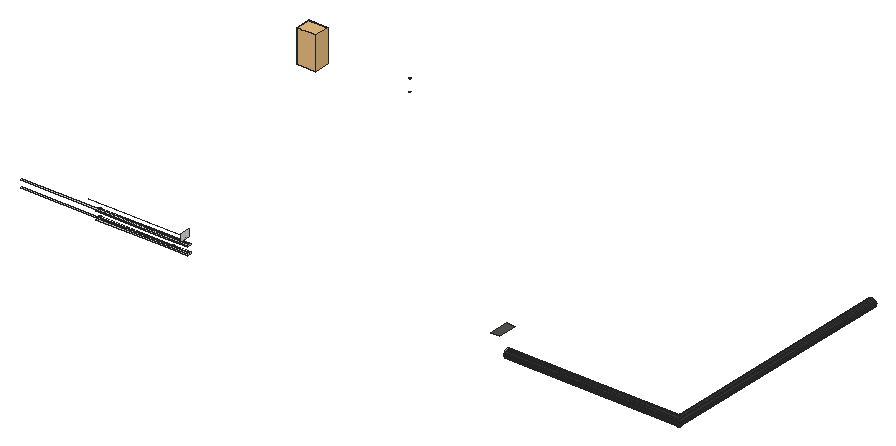
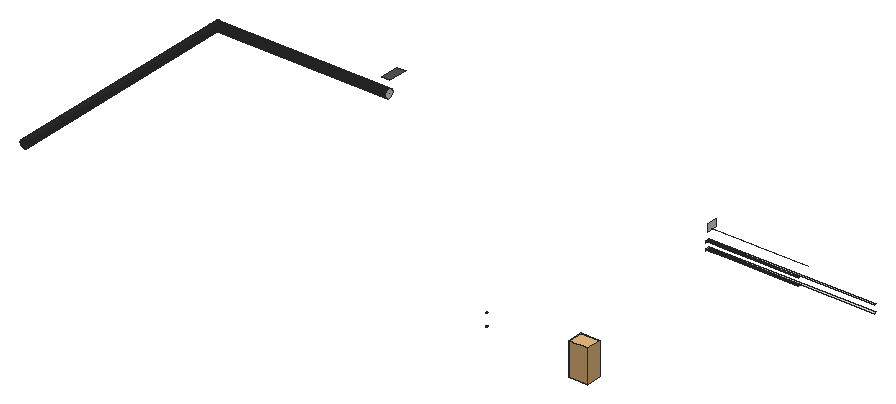
# SketchUp Ruby script. Lengths in inches.
U = 1.inch
M = Sketchup.active_model
def pt(a) = Geom::Point3d.new(a.map { |v| v * U })
def face(e, loops, mat)
  f = e.add_face(loops[0].map { |a| pt(a) })
  loops[1..].each { |l| e.add_face(l.map { |a| pt(a) }).erase! }
  f.material = f.back_material = mat if mat
  f
end
# faces: each face lists its corners as indices into pts; further lists are holes
def faces(e, pts, list, mat = nil) = list.each { |f| face(e, (f[0].is_a?(Array) ? f : [f]).map { |l| l.map { |i| pts[i] } }, mat) }
# xy, xz, yz: faces in a plane at the given z, y or x. An outline is a flat list of corners, or four numbers for a rectangle; further outlines are holes
def ring(l) = l.size == 4 ? [[l[0], l[1]], [l[2], l[1]], [l[2], l[3]], [l[0], l[3]]] : l.each_slice(2).to_a
def flat(e, list, mat, &to3) = list.each { |f| face(e, (f[0].is_a?(Array) ? f : [f]).map { |l| ring(l).map { |u, v| to3.(u, v) } }, mat) }
def xy(e, z, list, mat = nil) = flat(e, list, mat) { |x, y| [x, y, z] }
def xz(e, y, list, mat = nil) = flat(e, list, mat) { |x, z| [x, y, z] }
def yz(e, x, list, mat = nil) = flat(e, list, mat) { |y, z| [x, y, z] }
def lines(e, pts, list) = list.each { |a, b| e.add_line(pt(pts[a]), pt(pts[b])) }
# prism: a flat outline (further loops are holes) pulled along v
def prism(e, loops, v, mat = nil)
  f = face(e, loops, mat); d = Geom::Vector3d.new(v.map { |x| x * U })
  f.pushpull(f.normal.samedirection?(d) ? d.length : -d.length)
end
def box(e, o, s, mat = nil) = prism(e, [[o, [o[0] + s[0], o[1], o[2]], [o[0] + s[0], o[1] + s[1], o[2]], [o[0], o[1] + s[1], o[2]]]], [0, 0, s[2]], mat)
def at(x, y, z, deg = 0) = Geom::Transformation.translation(pt([x, y, z])) * Geom::Transformation.rotation(ORIGIN, Z_AXIS, deg.degrees)
def axes(o, x, y, z) = Geom::Transformation.new([*x, 0, *y, 0, *z, 0, *pt(o).to_a, 1])
def part(name) = M.definitions.add(name)
# library, detail: a bought-in or finely detailed component or shape, given as its bounding box
def library(name, o, s) = part(name).tap { |d| box(d.entities, o, s) }
def detail(e, o, s) = box(e.add_group.entities, o, s)
def put(e, d, t, mat = nil) = e.add_instance(d, t).tap { |i| i.material = mat if mat }
def group(e, t, mat = nil) = e.add_group.tap { |g| g.transformation = t; g.material = mat if mat }.entities
root = M.entities
M.materials.add("Generic\#2").color = [87, 84, 84]
M.materials.add("Material \#1").color = [140, 140, 140]
M.materials.add("[Color M07]").color = [58, 58, 58]
c1 = library("3DGeom~3_Defintion",[-83.33,-500,-350],[620.1,1000,533.33])
xy(root,150.7492,[[359.1551,130.1924,378.845,130.8174],[378.845,130.1924,383.845,130.8174]])
xy(root,151.1867,[[338.8426,130.1924,383.845,130.8174]])
xy(root,152.7492,[[359.1551,130.1924,378.845,130.8174],[378.845,130.1924,383.845,130.8174]])
xy(root,153.1867,[[338.8426,130.1924,383.845,130.8174]])
xy(root,157.4036,[[474.6154,129.427,474.7771,129.4483,474.9279,129.5107,475.0573,129.6101,475.1566,129.7395,475.2191,129.8903,475.2404,130.052,475.2191,130.2138,475.1566,130.3645,475.0573,130.494,474.9279,130.5933,474.7771,130.6557,474.6154,130.677,474.4536,130.6557,474.3029,130.5933,474.1734,130.494,474.0741,130.3645,474.0117,130.2138,473.9904,130.052,474.0117,129.8903,474.0741,129.7395,474.1734,129.6101,474.3029,129.5107,474.4536,129.4483],[490.9904,129.427,491.1521,129.4483,491.3029,129.5107,491.4323,129.6101,491.5316,129.7395,491.5941,129.8903,491.6154,130.052,491.5941,130.2138,491.5316,130.3645,491.4323,130.494,491.3029,130.5933,491.1521,130.6557,490.9904,130.677,490.8286,130.6557,490.6779,130.5933,490.5484,130.494,490.4491,130.3645,490.3867,130.2138,490.3654,130.052,490.3867,129.8903,490.4491,129.7395,490.5484,129.6101,490.6779,129.5107,490.8286,129.4483],[507.3654,129.427,507.5271,129.4483,507.6779,129.5107,507.8073,129.6101,507.9066,129.7395,507.9691,129.8903,507.9904,130.052,507.9691,130.2138,507.9066,130.3645,507.8073,130.494,507.6779,130.5933,507.5271,130.6557,507.3654,130.677,507.2036,130.6557,507.0529,130.5933,506.9234,130.494,506.8241,130.3645,506.7617,130.2138,506.7404,130.052,506.7617,129.8903,506.8241,129.7395,506.9234,129.6101,507.0529,129.5107,507.2036,129.4483],[516.5428,139.9993,516.7046,140.0206,516.8553,140.0831,516.9848,140.1824,517.0841,140.3118,517.1465,140.4626,517.1678,140.6243,517.1465,140.7861,517.0841,140.9368,516.9848,141.0663,516.8553,141.1656,516.7046,141.228,516.5428,141.2493,516.3811,141.228,516.2303,141.1656,516.1009,141.0663,516.0016,140.9368,515.9391,140.7861,515.9178,140.6243,515.9391,140.4626,516.0016,140.3118,516.1009,140.1824,516.2303,140.0831,516.3811,140.0206],[516.5428,151.8743,516.7046,151.8956,516.8553,151.9581,516.9848,152.0574,517.0841,152.1868,517.1465,152.3376,517.1678,152.4993,517.1465,152.6611,517.0841,152.8118,516.9848,152.9413,516.8553,153.0406,516.7046,153.103,516.5428,153.1243,516.3811,153.103,516.2303,153.0406,516.1009,152.9413,516.0016,152.8118,515.9391,152.6611,515.9178,152.4993,515.9391,152.3376,516.0016,152.1868,516.1009,152.0574,516.2303,151.9581,516.3811,151.8956],
  [516.5428,163.7493,516.7046,163.7706,516.8553,163.8331,516.9848,163.9324,517.0841,164.0618,517.1465,164.2126,517.1678,164.3743,517.1465,164.5361,517.0841,164.6868,516.9848,164.8163,516.8553,164.9156,516.7046,164.978,516.5428,164.9993,516.3811,164.978,516.2303,164.9156,516.1009,164.8163,516.0016,164.6868,515.9391,164.5361,515.9178,164.3743,515.9391,164.2126,516.0016,164.0618,516.1009,163.9324,516.2303,163.8331,516.3811,163.7706],[516.5428,175.6243,516.7046,175.6456,516.8553,175.7081,516.9848,175.8074,517.0841,175.9368,517.1465,176.0876,517.1678,176.2493,517.1465,176.4111,517.0841,176.5618,516.9848,176.6913,516.8553,176.7906,516.7046,176.853,516.5428,176.8743,516.3811,176.853,516.2303,176.7906,516.1009,176.6913,516.0016,176.5618,515.9391,176.4111,515.9178,176.2493,515.9391,176.0876,516.0016,175.9368,516.1009,175.8074,516.2303,175.7081,516.3811,175.6456]])
xy(root,161.0965,[[388.0139,199.7772,387.9576,199.7957,387.9662,199.8092],[388.0139,199.7772,387.9662,199.8092,388.0169,199.7926],[388.0139,199.7772,388.0169,199.7926,388.0739,199.7772],[388.0739,199.7772,388.0169,199.7926,388.0709,199.7926],[388.0739,199.7772,388.0709,199.7926,388.1303,199.7957],
  [388.0709,199.7926,388.1216,199.8092,388.1303,199.7957],[387.9576,199.7957,387.9116,199.8305,387.9249,199.8405],[387.9576,199.7957,387.9249,199.8405,387.9662,199.8092],[388.1303,199.7957,388.1216,199.8092,388.1762,199.8305],[388.1216,199.8092,388.163,199.8405,388.1762,199.8305],
  [387.9116,199.8305,387.8817,199.8772,387.8979,199.8826],[387.9116,199.8305,387.8979,199.8826,387.9249,199.8405],[388.1762,199.8305,388.163,199.8405,388.2062,199.8772],[388.163,199.8405,388.19,199.8826,388.2062,199.8772],[387.8817,199.8772,387.8712,199.9305,387.8885,199.9305],
  [387.8817,199.8772,387.8885,199.9305,387.8979,199.8826],[388.2062,199.8772,388.19,199.8826,388.2166,199.9305],[388.19,199.8826,388.1993,199.9305,388.2166,199.9305],[387.8712,199.9305,387.8817,199.9837,387.8979,199.9783],[387.8712,199.9305,387.8979,199.9783,387.8885,199.9305],
  [388.1993,199.9305,388.19,199.9783,388.2062,199.9837],[388.1993,199.9305,388.2062,199.9837,388.2166,199.9305],[387.8979,199.9783,387.8817,199.9837,387.9249,200.0205],[388.19,199.9783,388.163,200.0205,388.1762,200.0305],[388.19,199.9783,388.1762,200.0305,388.2062,199.9837],
  [387.8817,199.9837,387.9116,200.0305,387.9249,200.0205],[387.9249,200.0205,387.9116,200.0305,387.9662,200.0517],[388.163,200.0205,388.1216,200.0517,388.1303,200.0652],[388.163,200.0205,388.1303,200.0652,388.1762,200.0305],[387.9116,200.0305,387.9576,200.0652,387.9662,200.0517],
  [387.9662,200.0517,387.9576,200.0652,388.0169,200.0683],[388.1216,200.0517,388.0709,200.0683,388.0739,200.0837],[388.1216,200.0517,388.0739,200.0837,388.1303,200.0652],[387.9576,200.0652,388.0139,200.0837,388.0169,200.0683],[388.0169,200.0683,388.0139,200.0837,388.0709,200.0683],
  [388.0709,200.0683,388.0139,200.0837,388.0739,200.0837]],"Material \#1")
xy(root,161.1112,[[388.0139,199.7772,388.0169,199.7926,387.9576,199.7957],[388.0139,199.7772,388.0709,199.7926,388.0169,199.7926],[388.0139,199.7772,388.0739,199.7772,388.0709,199.7926],[388.0739,199.7772,388.1216,199.8092,388.0709,199.7926],[388.0739,199.7772,388.1303,199.7957,388.1216,199.8092],
  [388.0169,199.7926,387.9662,199.8092,387.9576,199.7957],[387.9576,199.7957,387.9662,199.8092,387.9116,199.8305],[388.1303,199.7957,388.163,199.8405,388.1216,199.8092],[388.1303,199.7957,388.1762,199.8305,388.163,199.8405],[387.9662,199.8092,387.9249,199.8405,387.9116,199.8305],
  [387.9116,199.8305,387.9249,199.8405,387.8817,199.8772],[388.1762,199.8305,388.19,199.8826,388.163,199.8405],[388.1762,199.8305,388.2062,199.8772,388.19,199.8826],[387.9249,199.8405,387.8979,199.8826,387.8817,199.8772],[387.8817,199.8772,387.8979,199.8826,387.8712,199.9305],
  [388.2062,199.8772,388.1993,199.9305,388.19,199.8826],[388.2062,199.8772,388.2166,199.9305,388.1993,199.9305],[387.8979,199.8826,387.8885,199.9305,387.8712,199.9305],[387.8712,199.9305,387.8885,199.9305,387.8817,199.9837],[387.8885,199.9305,387.8979,199.9783,387.8817,199.9837],
  [388.1993,199.9305,388.2166,199.9305,388.19,199.9783],[388.2166,199.9305,388.2062,199.9837,388.19,199.9783],[387.8979,199.9783,387.9116,200.0305,387.8817,199.9837],[387.8979,199.9783,387.9249,200.0205,387.9116,200.0305],[388.19,199.9783,388.2062,199.9837,388.163,200.0205],
  [388.2062,199.9837,388.1762,200.0305,388.163,200.0205],[387.9249,200.0205,387.9576,200.0652,387.9116,200.0305],[387.9249,200.0205,387.9662,200.0517,387.9576,200.0652],[388.163,200.0205,388.1762,200.0305,388.1216,200.0517],[388.1762,200.0305,388.1303,200.0652,388.1216,200.0517],
  [387.9662,200.0517,388.0139,200.0837,387.9576,200.0652],[387.9662,200.0517,388.0169,200.0683,388.0139,200.0837],[388.1216,200.0517,388.1303,200.0652,388.0709,200.0683],[388.1303,200.0652,388.0739,200.0837,388.0709,200.0683],[388.0169,200.0683,388.0739,200.0837,388.0139,200.0837],
  [388.0169,200.0683,388.0709,200.0683,388.0739,200.0837]],"Material \#1")
xy(root,162.875,[[467.9144,127.4375,470.2894,132.5625]],"Generic\#2")
xy(root,164.4068,[[388.0139,199.7772,387.9576,199.7957,388.0169,199.7926],[388.0139,199.7772,388.0169,199.7926,388.0709,199.7926],[388.0139,199.7772,388.0709,199.7926,388.0739,199.7772],[388.0739,199.7772,388.0709,199.7926,388.1216,199.8092],[388.0739,199.7772,388.1216,199.8092,388.1303,199.7957],
  [388.0169,199.7926,387.9576,199.7957,387.9662,199.8092],[387.9576,199.7957,387.9116,199.8305,387.9662,199.8092],[388.1303,199.7957,388.1216,199.8092,388.163,199.8405],[388.1303,199.7957,388.163,199.8405,388.1762,199.8305],[387.9662,199.8092,387.9116,199.8305,387.9249,199.8405],
  [387.9116,199.8305,387.8817,199.8772,387.9249,199.8405],[388.1762,199.8305,388.163,199.8405,388.19,199.8826],[388.1762,199.8305,388.19,199.8826,388.2062,199.8772],[387.9249,199.8405,387.8817,199.8772,387.8979,199.8826],[387.8817,199.8772,387.8712,199.9305,387.8979,199.8826],
  [388.2062,199.8772,388.19,199.8826,388.1993,199.9305],[388.2062,199.8772,388.1993,199.9305,388.2166,199.9305],[387.8979,199.8826,387.8712,199.9305,387.8885,199.9305],[387.8712,199.9305,387.8817,199.9837,387.8885,199.9305],[387.8885,199.9305,387.8817,199.9837,387.8979,199.9783],
  [388.1993,199.9305,388.19,199.9783,388.2166,199.9305],[388.2166,199.9305,388.19,199.9783,388.2062,199.9837],[387.8979,199.9783,387.8817,199.9837,387.9116,200.0305],[387.8979,199.9783,387.9116,200.0305,387.9249,200.0205],[388.19,199.9783,388.163,200.0205,388.2062,199.9837],
  [388.2062,199.9837,388.163,200.0205,388.1762,200.0305],[387.9249,200.0205,387.9116,200.0305,387.9576,200.0652],[387.9249,200.0205,387.9576,200.0652,387.9662,200.0517],[388.163,200.0205,388.1216,200.0517,388.1762,200.0305],[388.1762,200.0305,388.1216,200.0517,388.1303,200.0652],
  [387.9662,200.0517,387.9576,200.0652,388.0139,200.0837],[387.9662,200.0517,388.0139,200.0837,388.0169,200.0683],[388.1216,200.0517,388.0709,200.0683,388.1303,200.0652],[388.1303,200.0652,388.0709,200.0683,388.0739,200.0837],[388.0169,200.0683,388.0139,200.0837,388.0739,200.0837],
  [388.0169,200.0683,388.0739,200.0837,388.0709,200.0683]],"Material \#1")
xy(root,164.4215,[[388.0139,199.7772,387.9662,199.8092,387.9576,199.7957],[388.0139,199.7772,388.0169,199.7926,387.9662,199.8092],[388.0139,199.7772,388.0739,199.7772,388.0169,199.7926],[388.0739,199.7772,388.0709,199.7926,388.0169,199.7926],[388.0739,199.7772,388.1303,199.7957,388.0709,199.7926],
  [388.0709,199.7926,388.1303,199.7957,388.1216,199.8092],[387.9576,199.7957,387.9249,199.8405,387.9116,199.8305],[387.9576,199.7957,387.9662,199.8092,387.9249,199.8405],[388.1303,199.7957,388.1762,199.8305,388.1216,199.8092],[388.1216,199.8092,388.1762,199.8305,388.163,199.8405],
  [387.9116,199.8305,387.8979,199.8826,387.8817,199.8772],[387.9116,199.8305,387.9249,199.8405,387.8979,199.8826],[388.1762,199.8305,388.2062,199.8772,388.163,199.8405],[388.163,199.8405,388.2062,199.8772,388.19,199.8826],[387.8817,199.8772,387.8885,199.9305,387.8712,199.9305],
  [387.8817,199.8772,387.8979,199.8826,387.8885,199.9305],[388.2062,199.8772,388.2166,199.9305,388.19,199.8826],[388.19,199.8826,388.2166,199.9305,388.1993,199.9305],[387.8712,199.9305,387.8885,199.9305,387.8979,199.9783],[387.8712,199.9305,387.8979,199.9783,387.8817,199.9837],
  [388.1993,199.9305,388.2062,199.9837,388.19,199.9783],[388.1993,199.9305,388.2166,199.9305,388.2062,199.9837],[387.8979,199.9783,387.9249,200.0205,387.8817,199.9837],[388.19,199.9783,388.1762,200.0305,388.163,200.0205],[388.19,199.9783,388.2062,199.9837,388.1762,200.0305],
  [387.8817,199.9837,387.9249,200.0205,387.9116,200.0305],[387.9249,200.0205,387.9662,200.0517,387.9116,200.0305],[388.163,200.0205,388.1303,200.0652,388.1216,200.0517],[388.163,200.0205,388.1762,200.0305,388.1303,200.0652],[387.9116,200.0305,387.9662,200.0517,387.9576,200.0652],
  [387.9662,200.0517,388.0169,200.0683,387.9576,200.0652],[388.1216,200.0517,388.0739,200.0837,388.0709,200.0683],[388.1216,200.0517,388.1303,200.0652,388.0739,200.0837],[387.9576,200.0652,388.0169,200.0683,388.0139,200.0837],[388.0169,200.0683,388.0709,200.0683,388.0139,200.0837],
  [388.0709,200.0683,388.0739,200.0837,388.0139,200.0837]],"Material \#1")
xz(root,130.8174,[[359.1551,151.0617,378.845,151.1867],[378.845,151.0617,383.845,151.1867],[359.1551,153.0617,378.845,153.1867],[378.845,153.0617,383.845,153.1867]])
xz(root,199.2771,[[359.5512,160.6354,359.6089,160.6496,359.5813,160.6391],[359.5512,160.6354,359.6536,160.6877,359.6089,160.6496],[359.6089,160.6496,359.6536,160.6877,359.6333,160.6661],[359.6536,160.6877,359.3896,161.1332,359.4217,161.099],[359.6536,160.6877,359.4172,161.0585,359.4149,161.0634],
  [359.6536,160.6877,359.4187,161.0533,359.4172,161.0585],[359.6536,160.6877,359.4197,161.0478,359.4187,161.0533],[359.6536,160.6877,359.4217,161.099,359.4601,161.073],[359.6536,160.6877,359.5037,161.0564,359.5512,161.0506],[359.6536,160.6877,359.5512,161.0506,359.6825,160.7751],
  [359.6536,160.6877,359.679,160.7431,359.6691,160.7137],[359.6536,160.6877,359.6825,160.7751,359.679,160.7431],[359.6825,160.7751,359.5512,161.0506,359.5987,161.0564],[359.6825,160.7751,359.5987,161.0564,359.6423,161.073],[359.6825,160.7751,359.6423,161.073,359.6808,161.099],
  [359.6825,160.7751,359.6808,161.099,359.6825,161.0421],[359.6825,161.0421,359.6808,161.099,359.6838,161.0538],[359.6825,161.0421,359.6838,161.0538,359.6828,161.0482],[359.6838,161.0538,359.6808,161.099,359.7129,161.1332],[359.6838,161.0538,359.6878,161.0638,359.6855,161.059],
  [359.6838,161.0538,359.7129,161.1332,359.6878,161.0638],[359.6878,161.0638,359.7129,161.1332,359.7374,161.1741],[359.6878,161.0638,359.7374,161.1741,359.7839,161.2381],[359.6878,161.0638,359.7839,161.2381,359.6907,161.0684],[359.6907,161.0684,359.7839,161.2381,359.6943,161.0727],
  [359.6943,161.0727,359.7385,161.1225,359.6984,161.0768],[359.6943,161.0727,359.7839,161.2381,359.7385,161.1225],[359.6984,161.0768,359.7385,161.1225,359.7197,161.0985],[359.7385,161.1225,359.7679,161.1767,359.7547,161.1486],[359.7385,161.1225,359.7839,161.2381,359.7679,161.1767],
  [359.7374,161.1741,359.753,161.2205,359.7839,161.2381],[359.7679,161.1767,359.7839,161.2381,359.7778,161.2066],[359.753,161.2205,359.7584,161.271,359.7839,161.2381],[359.7839,161.2381,359.7344,161.4272,359.7799,161.3283],[359.7839,161.2381,359.7374,161.3679,359.7344,161.4272],
  [359.7839,161.2381,359.753,161.3215,359.7374,161.3679],[359.7839,161.2381,359.7584,161.271,359.753,161.3215],[359.7839,161.2381,359.7799,161.3283,359.7861,161.271],[359.7799,161.3283,359.7344,161.4272,359.7622,161.3808],[359.7374,161.3679,359.7129,161.4088,359.7344,161.4272],
  [359.7129,161.4088,359.6808,161.443,359.7344,161.4272],[359.7344,161.4272,359.5512,161.5209,359.6545,161.4954],[359.7344,161.4272,359.6423,161.469,359.5512,161.5209],[359.7344,161.4272,359.6808,161.443,359.6423,161.469],[359.7344,161.4272,359.6545,161.4954,359.6981,161.4659],
  [359.6423,161.469,359.5987,161.4856,359.5512,161.5209],[359.5987,161.4856,359.5512,161.4915,359.5512,161.5209],[359.6545,161.4954,359.5512,161.5209,359.605,161.5143]],"Material \#1")
xz(root,199.3082,[[359.5512,158.424,359.5512,158.4351,359.658,158.4453],[359.5512,158.424,359.658,158.4453,359.6599,158.4344],[359.6599,158.4344,359.658,158.4453,359.7583,158.4746],[359.6599,158.4344,359.7583,158.4746,359.7619,158.4642],[359.7619,158.4642,359.7583,158.4746,359.8507,158.5213],
  [359.7619,158.4642,359.8507,158.5213,359.8559,158.5117],[359.8559,158.5117,359.8507,158.5213,359.9336,158.5836],[359.8559,158.5117,359.9336,158.5836,359.9403,158.5752],[359.9403,158.5752,359.9336,158.5836,360.0052,158.6599],[359.9403,158.5752,360.0052,158.6599,360.0131,158.6527],
  [359.5512,158.5959,359.5853,158.6102,359.5871,158.5993],[359.5871,158.5993,359.5853,158.6102,359.6176,158.6197],[359.5871,158.5993,359.6176,158.6197,359.6212,158.6093],[359.6212,158.6093,359.6176,158.6197,359.6473,158.6347],[359.6212,158.6093,359.6473,158.6347,359.6525,158.6251],
  [359.6525,158.6251,359.6473,158.6347,359.6738,158.6546],[359.6525,158.6251,359.6738,158.6546,359.6805,158.6462],[359.6805,158.6462,359.6738,158.6546,359.6967,158.679],[359.6805,158.6462,359.6967,158.679,359.7046,158.6719],[360.0131,158.6527,360.0052,158.6599,360.0638,158.748],
  [360.0131,158.6527,360.0638,158.748,360.0728,158.7424],[359.7046,158.6719,359.6967,158.679,359.7155,158.7072],[359.7046,158.6719,359.7155,158.7072,359.7244,158.7016],[359.7244,158.7016,359.7155,158.7072,359.7296,158.7388],[359.7244,158.7016,359.7296,158.7388,359.7393,158.735],
  [359.7393,158.735,359.7296,158.7388,359.7385,158.7732],[359.7393,158.735,359.7385,158.7732,359.7487,158.7712],[360.0728,158.7424,360.0638,158.748,360.1077,158.8463],[360.0728,158.7424,360.1077,158.8463,360.1175,158.8425],[359.7487,158.7712,359.7385,158.7732,359.7415,158.8094],
  [359.7487,158.7712,359.7415,158.8094,359.7519,158.8094],[359.7415,158.8094,359.7385,158.8456,359.7519,158.8094],[359.7519,158.8094,359.7385,158.8456,359.7487,158.8476],[360.1175,158.8425,360.1077,158.8463,360.1353,158.953],[360.1175,158.8425,360.1353,158.953,360.1455,158.951],
  [359.7385,158.8456,359.7296,158.88,359.7487,158.8476],[359.7487,158.8476,359.7296,158.88,359.7393,158.8838],[359.7296,158.88,359.7155,158.9116,359.7393,158.8838],[359.7393,158.8838,359.7155,158.9116,359.7244,158.9172],[359.7155,158.9116,359.6967,158.9398,359.7244,158.9172],
  [359.7244,158.9172,359.6967,158.9398,359.7046,158.9469],[359.6967,158.9398,359.6738,158.9642,359.7046,158.9469],[359.7046,158.9469,359.6738,158.9642,359.6805,158.9726],[360.1455,158.951,360.1353,158.953,360.1453,159.0712],[360.1455,158.951,360.1453,159.0712,360.1556,159.0707],
  [359.6738,158.9642,359.6473,158.9841,359.6805,158.9726],[359.6805,158.9726,359.6473,158.9841,359.6525,158.9937],[359.6473,158.9841,359.6176,158.9991,359.6525,158.9937],[359.6525,158.9937,359.6176,158.9991,359.6212,159.0095],[359.6176,158.9991,359.5853,159.0086,359.6212,159.0095],
  [359.5853,159.0086,359.5512,159.0118,359.5871,159.0195],[359.5853,159.0086,359.5871,159.0195,359.6212,159.0095],[360.1556,159.0707,360.1453,159.0712,360.1453,164.8283],[360.1556,159.0707,360.1453,164.8283,360.1453,166.4101],[360.1556,159.0707,360.1453,166.4101,360.1556,166.4106]],"Material \#1")
xz(root,199.5882,[[359.5512,160.6354,359.5813,160.6391,359.6089,160.6496],[359.4935,160.6496,359.6089,160.6496,359.679,160.7431],[359.6089,160.6496,359.6333,160.6661,359.6536,160.6877],[359.6089,160.6496,359.6536,160.6877,359.679,160.7431],[359.6536,160.6877,359.6691,160.7137,359.679,160.7431],
  [359.679,160.7431,359.6825,160.7751,359.4149,161.0634],[359.6825,160.7751,359.5512,161.0506,359.5037,161.0564],[359.6825,160.7751,359.5987,161.0564,359.5512,161.0506],[359.6825,160.7751,359.6825,161.0421,359.5987,161.0564],[359.6825,161.0421,359.6838,161.0538,359.5987,161.0564],
  [359.6825,161.0421,359.6828,161.0482,359.6838,161.0538],[359.6838,161.0538,359.6878,161.0638,359.5987,161.0564],[359.6838,161.0538,359.6855,161.059,359.6878,161.0638],[359.5987,161.0564,359.6878,161.0638,359.6423,161.073],[359.6878,161.0638,359.6808,161.099,359.6423,161.073],
  [359.6878,161.0638,359.7129,161.1332,359.6808,161.099],[359.6878,161.0638,359.6907,161.0684,359.7839,161.2381],[359.6878,161.0638,359.7839,161.2381,359.7129,161.1332],[359.6907,161.0684,359.6943,161.0727,359.7839,161.2381],[359.6943,161.0727,359.6984,161.0768,359.7385,161.1225],
  [359.6943,161.0727,359.7385,161.1225,359.7839,161.2381],[359.6984,161.0768,359.7197,161.0985,359.7385,161.1225],[359.7385,161.1225,359.7547,161.1486,359.7679,161.1767],[359.7385,161.1225,359.7679,161.1767,359.7839,161.2381],[359.7129,161.1332,359.7839,161.2381,359.7374,161.1741],
  [359.7374,161.1741,359.7839,161.2381,359.753,161.2205],[359.7679,161.1767,359.7778,161.2066,359.7839,161.2381],[359.753,161.2205,359.7839,161.2381,359.7584,161.271],[359.7839,161.2381,359.7344,161.4272,359.753,161.3215],[359.7839,161.2381,359.7799,161.3283,359.7344,161.4272],
  [359.7839,161.2381,359.753,161.3215,359.7584,161.271],[359.7839,161.2381,359.7861,161.271,359.7799,161.3283],[359.753,161.3215,359.7344,161.4272,359.7374,161.3679],[359.7799,161.3283,359.7622,161.3808,359.7344,161.4272],[359.7374,161.3679,359.7344,161.4272,359.7129,161.4088],
  [359.7129,161.4088,359.7344,161.4272,359.6808,161.443],[359.7344,161.4272,359.5512,161.5209,359.6423,161.469],[359.7344,161.4272,359.6545,161.4954,359.5512,161.5209],[359.7344,161.4272,359.6423,161.469,359.6808,161.443],[359.7344,161.4272,359.6981,161.4659,359.6545,161.4954],
  [359.6423,161.469,359.5512,161.5209,359.5987,161.4856],[359.5987,161.4856,359.5512,161.5209,359.5512,161.4915],[359.6545,161.4954,359.605,161.5143,359.5512,161.5209]],"Material \#1")
xz(root,200.8328,[[359.5512,160.6354,359.6089,160.6496,359.5813,160.6391],[359.4935,160.6496,359.679,160.7431,359.6089,160.6496],[359.6089,160.6496,359.6536,160.6877,359.6333,160.6661],[359.6089,160.6496,359.679,160.7431,359.6536,160.6877],[359.6536,160.6877,359.679,160.7431,359.6691,160.7137],
  [359.679,160.7431,359.4149,161.0634,359.6825,160.7751],[359.6825,160.7751,359.5037,161.0564,359.5512,161.0506],[359.6825,160.7751,359.5512,161.0506,359.5987,161.0564],[359.6825,160.7751,359.5987,161.0564,359.6825,161.0421],[359.6825,161.0421,359.5987,161.0564,359.6838,161.0538],
  [359.6825,161.0421,359.6838,161.0538,359.6828,161.0482],[359.6838,161.0538,359.5987,161.0564,359.6878,161.0638],[359.6838,161.0538,359.6878,161.0638,359.6855,161.059],[359.5987,161.0564,359.6423,161.073,359.6878,161.0638],[359.6878,161.0638,359.6423,161.073,359.6808,161.099],
  [359.6878,161.0638,359.6808,161.099,359.7129,161.1332],[359.6878,161.0638,359.7129,161.1332,359.7839,161.2381],[359.6878,161.0638,359.7839,161.2381,359.6907,161.0684],[359.6907,161.0684,359.7839,161.2381,359.6943,161.0727],[359.6943,161.0727,359.7385,161.1225,359.6984,161.0768],
  [359.6943,161.0727,359.7839,161.2381,359.7385,161.1225],[359.6984,161.0768,359.7385,161.1225,359.7197,161.0985],[359.7385,161.1225,359.7679,161.1767,359.7547,161.1486],[359.7385,161.1225,359.7839,161.2381,359.7679,161.1767],[359.7129,161.1332,359.7374,161.1741,359.7839,161.2381],
  [359.7374,161.1741,359.753,161.2205,359.7839,161.2381],[359.7679,161.1767,359.7839,161.2381,359.7778,161.2066],[359.753,161.2205,359.7584,161.271,359.7839,161.2381],[359.7839,161.2381,359.7344,161.4272,359.7799,161.3283],[359.7839,161.2381,359.753,161.3215,359.7344,161.4272],
  [359.7839,161.2381,359.7584,161.271,359.753,161.3215],[359.7839,161.2381,359.7799,161.3283,359.7861,161.271],[359.753,161.3215,359.7374,161.3679,359.7344,161.4272],[359.7799,161.3283,359.7344,161.4272,359.7622,161.3808],[359.7374,161.3679,359.7129,161.4088,359.7344,161.4272],
  [359.7129,161.4088,359.6808,161.443,359.7344,161.4272],[359.7344,161.4272,359.5512,161.5209,359.6545,161.4954],[359.7344,161.4272,359.6423,161.469,359.5512,161.5209],[359.7344,161.4272,359.6808,161.443,359.6423,161.469],[359.7344,161.4272,359.6545,161.4954,359.6981,161.4659],
  [359.6423,161.469,359.5987,161.4856,359.5512,161.5209],[359.5987,161.4856,359.5512,161.4915,359.5512,161.5209],[359.6545,161.4954,359.5512,161.5209,359.605,161.5143]],"Material \#1")
xz(root,201.1128,[[359.5512,158.424,359.658,158.4453,359.5512,158.4351],[359.5512,158.424,359.6599,158.4344,359.658,158.4453],[359.6599,158.4344,359.7583,158.4746,359.658,158.4453],[359.6599,158.4344,359.7619,158.4642,359.7583,158.4746],[359.7619,158.4642,359.8507,158.5213,359.7583,158.4746],
  [359.7619,158.4642,359.8559,158.5117,359.8507,158.5213],[359.8559,158.5117,359.9336,158.5836,359.8507,158.5213],[359.8559,158.5117,359.9403,158.5752,359.9336,158.5836],[359.9403,158.5752,360.0052,158.6599,359.9336,158.5836],[359.9403,158.5752,360.0131,158.6527,360.0052,158.6599],
  [359.5512,158.5959,359.5871,158.5993,359.5853,158.6102],[359.5871,158.5993,359.6176,158.6197,359.5853,158.6102],[359.5871,158.5993,359.6212,158.6093,359.6176,158.6197],[359.6212,158.6093,359.6473,158.6347,359.6176,158.6197],[359.6212,158.6093,359.6525,158.6251,359.6473,158.6347],
  [359.6525,158.6251,359.6738,158.6546,359.6473,158.6347],[359.6525,158.6251,359.6805,158.6462,359.6738,158.6546],[359.6805,158.6462,359.6967,158.679,359.6738,158.6546],[359.6805,158.6462,359.7046,158.6719,359.6967,158.679],[360.0131,158.6527,360.0638,158.748,360.0052,158.6599],
  [360.0131,158.6527,360.0728,158.7424,360.0638,158.748],[359.7046,158.6719,359.7155,158.7072,359.6967,158.679],[359.7046,158.6719,359.7244,158.7016,359.7155,158.7072],[359.7244,158.7016,359.7296,158.7388,359.7155,158.7072],[359.7244,158.7016,359.7393,158.735,359.7296,158.7388],
  [359.7393,158.735,359.7385,158.7732,359.7296,158.7388],[359.7393,158.735,359.7487,158.7712,359.7385,158.7732],[360.0728,158.7424,360.1077,158.8463,360.0638,158.748],[360.0728,158.7424,360.1175,158.8425,360.1077,158.8463],[359.7487,158.7712,359.7415,158.8094,359.7385,158.7732],
  [359.7487,158.7712,359.7519,158.8094,359.7415,158.8094],[359.7415,158.8094,359.7519,158.8094,359.7385,158.8456],[359.7519,158.8094,359.7487,158.8476,359.7385,158.8456],[360.1175,158.8425,360.1353,158.953,360.1077,158.8463],[360.1175,158.8425,360.1455,158.951,360.1353,158.953],
  [359.7385,158.8456,359.7487,158.8476,359.7296,158.88],[359.7487,158.8476,359.7393,158.8838,359.7296,158.88],[359.7296,158.88,359.7393,158.8838,359.7155,158.9116],[359.7393,158.8838,359.7244,158.9172,359.7155,158.9116],[359.7155,158.9116,359.7244,158.9172,359.6967,158.9398],
  [359.7244,158.9172,359.7046,158.9469,359.6967,158.9398],[359.6967,158.9398,359.7046,158.9469,359.6738,158.9642],[359.7046,158.9469,359.6805,158.9726,359.6738,158.9642],[360.1455,158.951,360.1453,159.0712,360.1353,158.953],[360.1455,158.951,360.1556,159.0707,360.1453,159.0712],
  [359.6738,158.9642,359.6805,158.9726,359.6473,158.9841],[359.6805,158.9726,359.6525,158.9937,359.6473,158.9841],[359.6473,158.9841,359.6525,158.9937,359.6176,158.9991],[359.6525,158.9937,359.6212,159.0095,359.6176,158.9991],[359.6176,158.9991,359.6212,159.0095,359.5853,159.0086],
  [359.5853,159.0086,359.5871,159.0195,359.5512,159.0118],[359.5853,159.0086,359.6212,159.0095,359.5871,159.0195],[360.1556,159.0707,360.1453,164.8283,360.1453,159.0712],[360.1556,159.0707,360.1453,166.4101,360.1453,164.8283],[360.1556,159.0707,360.1556,166.4106,360.1453,166.4101]],"Material \#1")
xz(root,201.1439,[[359.5512,160.6354,359.5813,160.6391,359.6089,160.6496],[359.5512,160.6354,359.6089,160.6496,359.6536,160.6877],[359.6089,160.6496,359.6333,160.6661,359.6536,160.6877],[359.6536,160.6877,359.5512,161.0506,359.5037,161.0564],[359.6536,160.6877,359.6825,160.7751,359.5512,161.0506],
  [359.6536,160.6877,359.6691,160.7137,359.679,160.7431],[359.6536,160.6877,359.679,160.7431,359.6825,160.7751],[359.6825,160.7751,359.5987,161.0564,359.5512,161.0506],[359.6825,160.7751,359.6423,161.073,359.5987,161.0564],[359.6825,160.7751,359.6808,161.099,359.6423,161.073],
  [359.6825,160.7751,359.6825,161.0421,359.6808,161.099],[359.6825,161.0421,359.6838,161.0538,359.6808,161.099],[359.6825,161.0421,359.6828,161.0482,359.6838,161.0538],[359.6838,161.0538,359.7129,161.1332,359.6808,161.099],[359.6838,161.0538,359.6855,161.059,359.6878,161.0638],
  [359.6838,161.0538,359.6878,161.0638,359.7129,161.1332],[359.6878,161.0638,359.6907,161.0684,359.7839,161.2381],[359.6878,161.0638,359.7374,161.1741,359.7129,161.1332],[359.6878,161.0638,359.7839,161.2381,359.7374,161.1741],[359.6907,161.0684,359.6943,161.0727,359.7839,161.2381],
  [359.6943,161.0727,359.6984,161.0768,359.7385,161.1225],[359.6943,161.0727,359.7385,161.1225,359.7839,161.2381],[359.6984,161.0768,359.7197,161.0985,359.7385,161.1225],[359.7385,161.1225,359.7547,161.1486,359.7679,161.1767],[359.7385,161.1225,359.7679,161.1767,359.7839,161.2381],
  [359.7374,161.1741,359.7839,161.2381,359.753,161.2205],[359.7679,161.1767,359.7778,161.2066,359.7839,161.2381],[359.753,161.2205,359.7839,161.2381,359.7584,161.271],[359.7839,161.2381,359.7344,161.4272,359.7374,161.3679],[359.7839,161.2381,359.7799,161.3283,359.7344,161.4272],
  [359.7839,161.2381,359.7374,161.3679,359.753,161.3215],[359.7839,161.2381,359.753,161.3215,359.7584,161.271],[359.7839,161.2381,359.7861,161.271,359.7799,161.3283],[359.7799,161.3283,359.7622,161.3808,359.7344,161.4272],[359.7374,161.3679,359.7344,161.4272,359.7129,161.4088],
  [359.7129,161.4088,359.7344,161.4272,359.6808,161.443],[359.7344,161.4272,359.5512,161.5209,359.6423,161.469],[359.7344,161.4272,359.6545,161.4954,359.5512,161.5209],[359.7344,161.4272,359.6423,161.469,359.6808,161.443],[359.7344,161.4272,359.6981,161.4659,359.6545,161.4954],
  [359.6423,161.469,359.5512,161.5209,359.5987,161.4856],[359.5987,161.4856,359.5512,161.5209,359.5512,161.4915],[359.6545,161.4954,359.605,161.5143,359.5512,161.5209]],"Material \#1")
yz(root,359.5715,[[199.2677,161.2049,199.5571,161.2049,199.5571,161.2306],[199.2677,161.2049,199.5571,161.2306,199.2677,161.2306],[200.8639,161.2049,201.1532,161.2049,200.8639,161.2306],[201.1532,161.2049,201.1532,161.2306,200.8639,161.2306]],"Material \#1")
yz(root,359.5765,[[199.2677,161.3078,199.5571,161.3078,199.5571,161.3555],[200.8639,161.3078,201.1532,161.3078,200.8639,161.3555]],"Material \#1")
yz(root,359.579,[[199.2677,161.2514,199.5571,161.2514,199.5571,161.2722],[199.2677,161.2514,199.5571,161.2722,199.2677,161.2722],[200.8639,161.2514,201.1532,161.2514,200.8639,161.2722],[201.1532,161.2514,201.1532,161.2722,200.8639,161.2722]],"Material \#1")
yz(root,383.845,[[131.3497,150.7247,131.3497,151.0372,131.3554,151.1621,130.8231,151.1865,130.8174,151.0617,130.8174,151.1867,130.1924,151.1867,130.1924,150.7492,130.8174,150.7492],[131.3497,152.7247,131.3497,153.0372,131.3554,153.1621,130.8231,153.1865,130.8174,153.0617,130.8174,153.1867,130.1924,153.1867,130.1924,152.7492,130.8174,152.7492],[128.022,155.0367,130.647,156.9742]])
yz(root,470.2894,[[129.8903,156.5826,129.6036,156.6203,129.3364,156.731,129.107,156.907,128.9309,157.1365,128.8203,157.4036,128.7825,157.6903,128.8203,157.977,128.9309,158.2442,129.107,158.4736,129.3364,158.6497,129.6036,158.7603,129.8903,158.7981,130.177,158.7603,130.4441,158.6497,130.6735,158.4736,130.8496,158.2442,130.9602,157.977,130.998,157.6903,130.9602,157.4036,130.8496,157.1365,130.6735,156.907,130.4441,156.731,130.177,156.6203]])
p = [[378.845,131.3497,151.0372],[359.1551,131.3497,151.0372],[359.1551,131.3554,151.1621],[378.845,131.3554,151.1621],[383.845,131.3497,151.0372],[383.845,131.3554,151.1621],
  [359.1551,130.8174,151.0617],[378.845,130.8174,151.0617],[378.845,130.8231,151.1865],[359.1551,130.8231,151.1865],[383.845,130.8174,151.0617],[383.845,130.8231,151.1865],
  [378.845,131.3497,153.0372],[359.1551,131.3497,153.0372],[359.1551,131.3554,153.1621],[378.845,131.3554,153.1621],[383.845,131.3497,153.0372],[383.845,131.3554,153.1621],
  [359.1551,130.8174,153.0617],[378.845,130.8174,153.0617],[378.845,130.8231,153.1865],[359.1551,130.8231,153.1865],[383.845,130.8174,153.0617],[383.845,130.8231,153.1865],
  [470.2894,129.3364,156.731],[470.2894,129.6036,156.6203],[516.9913,129.6036,156.6203],[517.2585,129.3364,156.731],[516.9913,131.125,156.6203],[516.9913,194.75,156.6203],
  [517.2585,194.75,156.731],[517.2585,131.125,156.731],[470.2894,129.8903,156.5826],[474.0117,129.8903,156.5826],[475.2191,129.8903,156.5826],[490.3867,129.8903,156.5826],
  [491.5941,129.8903,156.5826],[506.7617,129.8903,156.5826],[507.9691,129.8903,156.5826],[516.7046,129.8903,156.5826],[516.7046,176.853,156.5826],[516.7046,194.75,156.5826],
  [516.7046,131.125,156.5826],[516.7046,140.0206,156.5826],[516.7046,141.228,156.5826],[516.7046,151.8956,156.5826],[516.7046,153.103,156.5826],[516.7046,163.7706,156.5826],
  [516.7046,164.978,156.5826],[516.7046,175.6456,156.5826],[470.2894,130.177,156.6203],[516.4179,130.177,156.6203],[516.4179,131.125,156.6203],[516.4179,194.75,156.6203],
  [470.2894,130.4441,156.731],[516.1507,130.4441,156.731],[516.1507,131.125,156.731],[516.1507,194.75,156.731],[470.2894,129.107,156.907],[517.4879,129.107,156.907],
  [517.4879,194.75,156.907],[517.4879,131.125,156.907],[470.2894,130.6735,156.907],[515.9213,130.6735,156.907],[515.9213,131.125,156.907],[515.9213,194.75,156.907],
  [470.2894,128.9309,157.1365],[517.6639,128.9309,157.1365],[517.6639,194.75,157.1365],[517.6639,131.125,157.1365],[470.2894,130.8496,157.1365],[515.7453,130.8496,157.1365],
  [515.7453,131.125,157.1365],[515.7453,194.75,157.1365],[470.2894,128.8203,157.4036],[517.7746,128.8203,157.4036],[517.7746,194.75,157.4036],[517.7746,131.125,157.4036],
  [470.2894,130.9602,157.4036],[515.6346,130.9602,157.4036],[515.6346,131.125,157.4036],[515.6346,194.75,157.4036],[470.2894,128.7825,157.6903],[517.8123,128.7825,157.6903],
  [517.8123,194.75,157.6903],[517.8123,131.125,157.6903],[470.2894,130.998,157.6903],[515.5969,130.998,157.6903],[515.5969,131.125,157.6903],[515.5969,194.75,157.6903],
  [470.2894,128.8203,157.977],[517.7746,128.8203,157.977],[517.7746,194.75,157.977],[517.7746,131.125,157.977],[470.2894,130.9602,157.977],[515.6346,130.9602,157.977],
  [515.6346,131.125,157.977],[515.6346,194.75,157.977],[470.2894,128.9309,158.2442],[517.6639,128.9309,158.2442],[517.6639,194.75,158.2442],[517.6639,131.125,158.2442],
  [470.2894,130.8496,158.2442],[515.7453,130.8496,158.2442],[515.7453,131.125,158.2442],[515.7453,194.75,158.2442],[470.2894,129.107,158.4736],[517.4879,129.107,158.4736],
  [517.4879,194.75,158.4736],[517.4879,131.125,158.4736],[470.2894,130.6735,158.4736],[515.9213,130.6735,158.4736],[515.9213,131.125,158.4736],[515.9213,194.75,158.4736],
  [470.2894,129.3364,158.6497],[517.2585,129.3364,158.6497],[517.2585,194.75,158.6497],[517.2585,131.125,158.6497],[470.2894,130.4441,158.6497],[516.1507,130.4441,158.6497],
  [516.1507,131.125,158.6497],[516.1507,194.75,158.6497],[470.2894,129.6036,158.7603],[516.9913,129.6036,158.7603],[516.9913,194.75,158.7603],[516.9913,131.125,158.7603],
  [470.2894,130.177,158.7603],[516.4179,130.177,158.7603],[516.4179,131.125,158.7603],[516.4179,194.75,158.7603],[470.2894,129.8903,158.7981],[516.7046,129.8903,158.7981],
  [516.7046,194.75,158.7981],[516.7046,131.125,158.7981],[359.5641,199.2677,161.1498],[359.5615,199.5571,161.1461],[359.5667,199.5571,161.1535],[359.5641,199.2677,161.1498],
  [359.5667,199.5571,161.1535],[359.5667,199.5571,161.17],[359.5641,199.2677,161.1736],[359.5615,199.5571,161.1461],[359.5641,199.2677,161.1498],[359.5715,199.2677,161.1241],
  [359.5715,199.2677,161.1241],[359.5715,199.5571,161.1241],[359.5615,199.5571,161.1461],[359.5641,201.1532,161.1498],[359.5641,201.1532,161.1736],[359.5667,200.8639,161.17],
  [359.5667,200.8639,161.1535],[359.5715,201.1532,161.1241],[359.5641,201.1532,161.1498],[359.5615,200.8639,161.1461],[359.5615,200.8639,161.1461],[359.5715,200.8639,161.1241],
  [359.5715,201.1532,161.1241],[359.5641,199.2677,161.1736],[359.5667,199.5571,161.17],[359.5615,199.5571,161.1773],[359.5641,199.2677,161.1736],[359.5615,199.5571,161.1773],
  [359.5715,199.5571,161.2049],[359.5715,199.5571,161.2049],[359.5715,199.2677,161.2049],[359.5641,199.2677,161.1736],[359.5715,199.2677,161.2306],[359.5715,199.5571,161.2306],
  [359.579,199.5571,161.2514],[359.579,199.5571,161.2514],[359.579,199.2677,161.2514],[359.5715,199.2677,161.2306],[359.5715,200.8639,161.2049],[359.5615,200.8639,161.1773],
  [359.5641,201.1532,161.1736],[359.5641,201.1532,161.1736],[359.5715,201.1532,161.2049],[359.5715,200.8639,161.2049],[359.5715,201.1532,161.2306],[359.579,201.1532,161.2514],
  [359.579,200.8639,161.2514],[359.5715,200.8639,161.2306],[359.5715,199.2677,161.2931],[359.5715,199.5571,161.2931],[359.5765,199.5571,161.3078],[359.5715,199.5571,161.2931],
  [359.5715,199.2677,161.2931],[359.579,199.2677,161.2722],[359.5765,199.5571,161.3078],[359.5765,199.2677,161.3078],[359.5715,199.2677,161.2931],[359.5765,199.5571,161.3555],
  [359.5738,199.2677,161.3645],[359.5765,199.2677,161.3078],[359.579,199.2677,161.2722],[359.579,199.5571,161.2722],[359.5715,199.5571,161.2931],[359.5765,200.8639,161.3078],
  [359.5715,200.8639,161.2931],[359.5715,201.1532,161.2931],[359.579,201.1532,161.2722],[359.5715,201.1532,161.2931],[359.5715,200.8639,161.2931],[359.5715,201.1532,161.2931],
  [359.5765,201.1532,161.3078],[359.5765,200.8639,161.3078],[359.5765,201.1532,161.3078],[359.5738,201.1532,161.3645],[359.5765,200.8639,161.3555],[359.5715,200.8639,161.2931],
  [359.579,200.8639,161.2722],[359.579,201.1532,161.2722],[359.5738,199.2677,161.3645],[359.5765,199.5571,161.3702],[359.5765,199.5571,161.418],[359.5765,199.5571,161.418],
  [359.5765,199.2677,161.418],[359.5738,199.2677,161.3645],[359.5765,200.8639,161.418],[359.5765,200.8639,161.3702],[359.5738,201.1532,161.3645],[359.5738,201.1532,161.3645],
  [359.5765,201.1532,161.418],[359.5765,200.8639,161.418],[470.2894,129.8903,157.6903],[516.7046,129.8903,157.6903],[516.7046,194.75,157.6903],[516.7046,131.125,157.6903],
  [376.6602,129.6447,155.4651],[382.9102,129.6447,155.4651],[357.5352,129.6447,155.4651],[383.845,129.6447,155.4651],[383.845,130.9647,152.8984],[378.845,130.9647,152.8984],
  [359.1551,130.9647,152.8984],[383.845,130.9647,150.8984],[378.845,130.9647,150.8984],[359.1551,130.9647,150.8984]]
faces(root,p,[[0,1,2,3],[4,0,3,5],[6,7,8,9],[7,10,11,8],[12,13,14,15],[16,12,15,17],[18,19,20,21],[19,22,23,20]])
faces(root,p,[[24,25,26,27],[28,29,30,31,27,26],[25,32,33,34,35,36,37,38,39,26],[40,41,29,28,26,39,42,43,44,45,46,47,48,49],[32,50,51,39,38,37,36,35,34,33],[39,51,52,53,41,40,49,48,47,46,45,44,43,42],[50,54,55,51],[56,57,53,52,51,55],
  [58,24,27,59],[31,30,60,61,59,27],[54,62,63,55],[55,63,64,65,57,56],[66,58,59,67],[61,60,68,69,67,59],[62,70,71,63],[63,71,72,73,65,64],
  [74,66,67,75],[69,68,76,77,75,67],[70,78,79,71],[71,79,80,81,73,72],[82,74,75,83],[77,76,84,85,83,75],[78,86,87,79],[79,87,88,89,81,80],
  [90,82,83,91],[85,84,92,93,91,83],[86,94,95,87],[96,97,89,88,87,95],[98,90,91,99],[93,92,100,101,99,91],[94,102,103,95],[95,103,104,105,97,96],
  [106,98,99,107],[101,100,108,109,107,99],[102,110,111,103],[103,111,112,113,105,104],[114,106,107,115],[109,108,116,117,115,107],[110,118,119,111],[111,119,120,121,113,112],
  [122,114,115,123],[117,116,124,125,123,115],[118,126,127,119],[119,127,128,129,121,120],[130,122,123,131],[125,124,132,133,131,123],[126,130,131,127],[133,132,129,128,127,131]],"[Color M07]")
faces(root,p,[[134,135,136],[137,138,139],[139,140,137],[141,142,143],[144,145,146],[147,148,149],[149,150,147],[151,152,153],
  [154,155,156],[157,158,159],[160,161,162],[163,164,165],[166,167,168],[169,170,171],[172,173,174],[175,176,177],
  [178,179,180],[180,181,178],[182,183,184],[185,186,187],[188,189,190],[191,192,193],[194,195,196],[197,198,199],
  [200,201,202],[203,204,205],[206,207,208],[209,210,211],[212,213,214],[215,216,217],[218,219,220],[221,222,223]],"Material \#1")
lines(root,p,[[224,225],[226,227],[227,225],[228,229],[228,230],[229,231],[232,233],[233,234],[235,236],[236,237]])
put(root,c1,axes([359.55,200.83,162.74],[0.00829,0,0],[0,0,0.00882],[0,0.00747,0]),"Material \#1")
